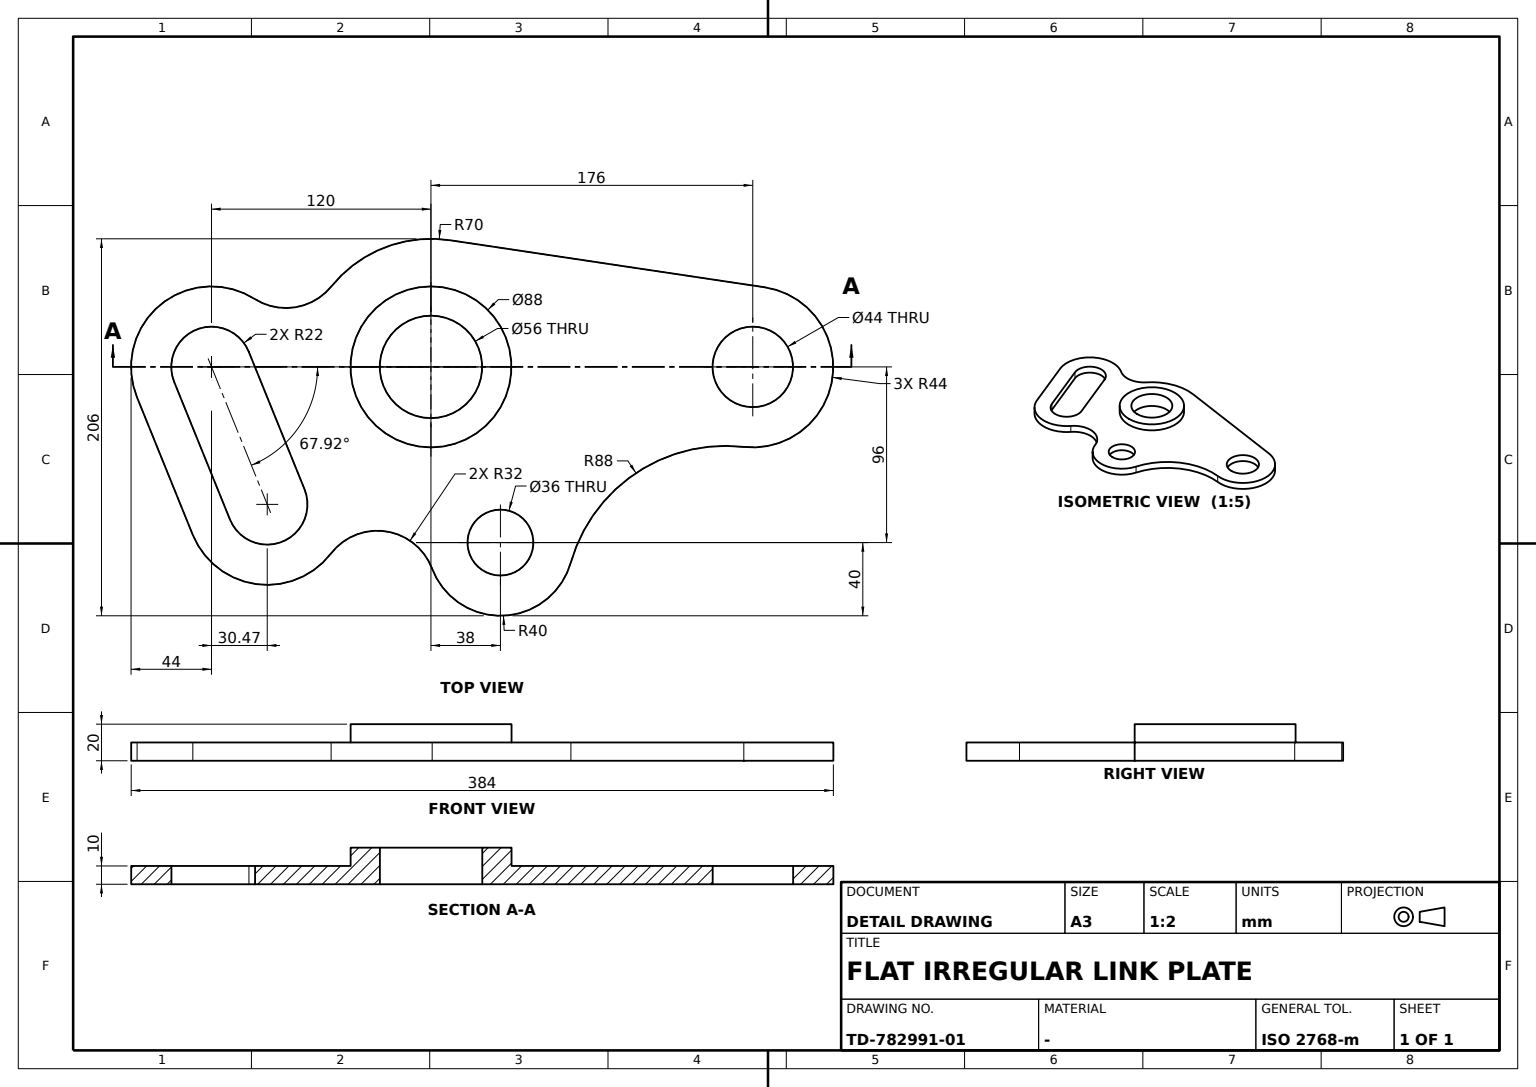
ISO-10303-21;
HEADER;
FILE_DESCRIPTION((''),'2;1');
FILE_NAME('','',(''),(''),'','','');
FILE_SCHEMA(('AUTOMOTIVE_DESIGN'));
ENDSEC;
DATA;
#1=APPLICATION_CONTEXT('');
#2=PRODUCT_CONTEXT('',#1,'mechanical');
#3=PRODUCT('','','',(#2));
#4=PRODUCT_DEFINITION_FORMATION('','',#3);
#5=PRODUCT_DEFINITION_CONTEXT('',#1,'design');
#6=PRODUCT_DEFINITION('','',#4,#5);
#7=PRODUCT_DEFINITION_SHAPE('','',#6);
#8=(LENGTH_UNIT()NAMED_UNIT(*)SI_UNIT(.MILLI.,.METRE.));
#9=(NAMED_UNIT(*)PLANE_ANGLE_UNIT()SI_UNIT($,.RADIAN.));
#10=(NAMED_UNIT(*)SI_UNIT($,.STERADIAN.)SOLID_ANGLE_UNIT());
#11=UNCERTAINTY_MEASURE_WITH_UNIT(LENGTH_MEASURE(0.005),#8,'distance_accuracy_value','');
#12=(GEOMETRIC_REPRESENTATION_CONTEXT(3)GLOBAL_UNCERTAINTY_ASSIGNED_CONTEXT((#11))GLOBAL_UNIT_ASSIGNED_CONTEXT((#8,#9,#10))REPRESENTATION_CONTEXT('',''));
#13=CARTESIAN_POINT('',(-43.517238,182.5,0.));
#14=VERTEX_POINT('',#13);
#15=CARTESIAN_POINT('',(-43.517238,182.5,-10.));
#16=VERTEX_POINT('',#15);
#17=CARTESIAN_POINT('',(-43.517238,182.5,-5.));
#18=DIRECTION('',(0.,0.,1.));
#19=VECTOR('',#18,1000.);
#20=LINE('',#17,#19);
#21=EDGE_CURVE('',#14,#16,#20,.F.);
#22=ORIENTED_EDGE('',*,*,#21,.F.);
#23=CARTESIAN_POINT('',(43.717954,171.026016,0.));
#24=VERTEX_POINT('',#23);
#25=CARTESIAN_POINT('',(0.,176.,0.));
#26=DIRECTION('',(1.,0.,0.));
#27=AXIS2_PLACEMENT_3D('',#25,#18,#26);
#28=CIRCLE('',#27,44.);
#29=EDGE_CURVE('',#24,#14,#28,.T.);
#30=ORIENTED_EDGE('',*,*,#29,.F.);
#31=CARTESIAN_POINT('',(43.717954,171.026016,-10.));
#32=VERTEX_POINT('',#31);
#33=CARTESIAN_POINT('',(43.717954,171.026016,-5.));
#34=LINE('',#33,#19);
#35=EDGE_CURVE('',#24,#32,#34,.F.);
#36=ORIENTED_EDGE('',*,*,#35,.T.);
#37=CARTESIAN_POINT('',(0.,176.,-10.));
#38=AXIS2_PLACEMENT_3D('',#37,#18,#26);
#39=CIRCLE('',#38,44.);
#40=EDGE_CURVE('',#32,#16,#39,.T.);
#41=ORIENTED_EDGE('',*,*,#40,.T.);
#42=EDGE_LOOP('',(#22,#30,#36,#41));
#43=FACE_BOUND('',#42,.T.);
#44=CARTESIAN_POINT('',(0.,176.,-5.));
#45=AXIS2_PLACEMENT_3D('',#44,#18,#26);
#46=CYLINDRICAL_SURFACE('',#45,44.);
#47=ADVANCED_FACE('',(#43),#46,.T.);
#48=CARTESIAN_POINT('',(28.,0.,-10.));
#49=VERTEX_POINT('',#48);
#50=CARTESIAN_POINT('',(0.,0.,-10.));
#51=AXIS2_PLACEMENT_3D('',#50,#18,#26);
#52=CIRCLE('',#51,28.);
#53=EDGE_CURVE('',#49,#49,#52,.T.);
#54=ORIENTED_EDGE('',*,*,#53,.T.);
#55=EDGE_LOOP('',(#54));
#56=FACE_BOUND('',#55,.T.);
#57=CARTESIAN_POINT('',(22.,176.,-10.));
#58=VERTEX_POINT('',#57);
#59=CIRCLE('',#38,22.);
#60=EDGE_CURVE('',#58,#58,#59,.T.);
#61=ORIENTED_EDGE('',*,*,#60,.T.);
#62=EDGE_LOOP('',(#61));
#63=FACE_BOUND('',#62,.T.);
#64=CARTESIAN_POINT('',(-8.270016,-99.613563,-10.));
#65=VERTEX_POINT('',#64);
#66=CARTESIAN_POINT('',(66.851293,-69.139653,-10.));
#67=VERTEX_POINT('',#66);
#68=DIRECTION('',(0.926656248,0.375909827,0.));
#69=VECTOR('',#68,1000.);
#70=LINE('',#64,#69);
#71=EDGE_CURVE('',#65,#67,#70,.T.);
#72=ORIENTED_EDGE('',*,*,#71,.F.);
#73=CARTESIAN_POINT('',(8.270016,-140.386437,-10.));
#74=VERTEX_POINT('',#73);
#75=CARTESIAN_POINT('',(0.,-120.,-10.));
#76=AXIS2_PLACEMENT_3D('',#75,#18,#26);
#77=CIRCLE('',#76,22.);
#78=EDGE_CURVE('',#65,#74,#77,.T.);
#79=ORIENTED_EDGE('',*,*,#78,.T.);
#80=CARTESIAN_POINT('',(83.391326,-109.912528,-10.));
#81=VERTEX_POINT('',#80);
#82=DIRECTION('',(-0.926656248,-0.375909827,0.));
#83=VECTOR('',#82,1000.);
#84=LINE('',#80,#83);
#85=EDGE_CURVE('',#81,#74,#84,.T.);
#86=ORIENTED_EDGE('',*,*,#85,.F.);
#87=CARTESIAN_POINT('',(75.12131,-89.526091,-10.));
#88=AXIS2_PLACEMENT_3D('',#87,#18,#26);
#89=CIRCLE('',#88,22.);
#90=EDGE_CURVE('',#81,#67,#89,.T.);
#91=ORIENTED_EDGE('',*,*,#90,.T.);
#92=EDGE_LOOP('',(#72,#79,#86,#91));
#93=FACE_BOUND('',#92,.T.);
#94=CARTESIAN_POINT('',(-69.231969,10.340909,-10.));
#95=VERTEX_POINT('',#94);
#96=DIRECTION('',(0.147727273,0.989028136,0.));
#97=VECTOR('',#96,1000.);
#98=LINE('',#94,#97);
#99=EDGE_CURVE('',#95,#16,#98,.T.);
#100=ORIENTED_EDGE('',*,*,#99,.T.);
#101=ORIENTED_EDGE('',*,*,#40,.F.);
#102=CARTESIAN_POINT('',(106.985582,76.46189,-10.));
#103=VERTEX_POINT('',#102);
#104=CARTESIAN_POINT('',(131.153861,161.078049,-10.));
#105=AXIS2_PLACEMENT_3D('',#104,#18,#26);
#106=CIRCLE('',#105,88.);
#107=EDGE_CURVE('',#32,#103,#106,.T.);
#108=ORIENTED_EDGE('',*,*,#107,.T.);
#109=CARTESIAN_POINT('',(110.17399,0.595482,-10.));
#110=VERTEX_POINT('',#109);
#111=CARTESIAN_POINT('',(96.,38.,-10.));
#112=AXIS2_PLACEMENT_3D('',#111,#18,#26);
#113=CIRCLE('',#112,40.);
#114=EDGE_CURVE('',#110,#103,#113,.T.);
#115=ORIENTED_EDGE('',*,*,#114,.F.);
#116=CARTESIAN_POINT('',(101.979763,-54.674642,-10.));
#117=VERTEX_POINT('',#116);
#118=CARTESIAN_POINT('',(121.513183,-29.328133,-10.));
#119=AXIS2_PLACEMENT_3D('',#118,#18,#26);
#120=CIRCLE('',#119,32.);
#121=EDGE_CURVE('',#110,#117,#120,.T.);
#122=ORIENTED_EDGE('',*,*,#121,.T.);
#123=CARTESIAN_POINT('',(91.661342,-130.298966,-10.));
#124=VERTEX_POINT('',#123);
#125=CIRCLE('',#88,44.);
#126=EDGE_CURVE('',#124,#117,#125,.T.);
#127=ORIENTED_EDGE('',*,*,#126,.F.);
#128=CARTESIAN_POINT('',(16.540032,-160.772875,-10.));
#129=VERTEX_POINT('',#128);
#130=LINE('',#123,#83);
#131=EDGE_CURVE('',#124,#129,#130,.T.);
#132=ORIENTED_EDGE('',*,*,#131,.T.);
#133=CARTESIAN_POINT('',(-37.152695,-96.427193,-10.));
#134=VERTEX_POINT('',#133);
#135=CIRCLE('',#76,44.);
#136=EDGE_CURVE('',#134,#129,#135,.T.);
#137=ORIENTED_EDGE('',*,*,#136,.F.);
#138=CARTESIAN_POINT('',(-44.040183,-54.410131,-10.));
#139=VERTEX_POINT('',#138);
#140=CARTESIAN_POINT('',(-64.172837,-79.283333,-10.));
#141=AXIS2_PLACEMENT_3D('',#140,#18,#26);
#142=CIRCLE('',#141,32.);
#143=EDGE_CURVE('',#134,#139,#142,.T.);
#144=ORIENTED_EDGE('',*,*,#143,.T.);
#145=CIRCLE('',#51,70.);
#146=EDGE_CURVE('',#95,#139,#145,.T.);
#147=ORIENTED_EDGE('',*,*,#146,.F.);
#148=EDGE_LOOP('',(#100,#101,#108,#115,#122,#127,#132,#137,#144,#147));
#149=FACE_BOUND('',#148,.T.);
#150=CARTESIAN_POINT('',(114.,38.,-10.));
#151=VERTEX_POINT('',#150);
#152=CIRCLE('',#112,18.);
#153=EDGE_CURVE('',#151,#151,#152,.T.);
#154=ORIENTED_EDGE('',*,*,#153,.T.);
#155=EDGE_LOOP('',(#154));
#156=FACE_BOUND('',#155,.T.);
#157=PLANE('',#51);
#158=ADVANCED_FACE('',(#56,#63,#93,#149,#156),#157,.F.);
#159=ORIENTED_EDGE('',*,*,#60,.F.);
#160=EDGE_LOOP('',(#159));
#161=FACE_BOUND('',#160,.T.);
#162=CARTESIAN_POINT('',(22.,176.,0.));
#163=VERTEX_POINT('',#162);
#164=CIRCLE('',#27,22.);
#165=EDGE_CURVE('',#163,#163,#164,.T.);
#166=ORIENTED_EDGE('',*,*,#165,.T.);
#167=EDGE_LOOP('',(#166));
#168=FACE_BOUND('',#167,.T.);
#169=CYLINDRICAL_SURFACE('',#45,22.);
#170=ADVANCED_FACE('',(#161,#168),#169,.F.);
#171=CARTESIAN_POINT('',(28.,0.,10.));
#172=VERTEX_POINT('',#171);
#173=CARTESIAN_POINT('',(0.,0.,10.));
#174=AXIS2_PLACEMENT_3D('',#173,#18,#26);
#175=CIRCLE('',#174,28.);
#176=EDGE_CURVE('',#172,#172,#175,.T.);
#177=ORIENTED_EDGE('',*,*,#176,.T.);
#178=EDGE_LOOP('',(#177));
#179=FACE_BOUND('',#178,.T.);
#180=ORIENTED_EDGE('',*,*,#53,.F.);
#181=EDGE_LOOP('',(#180));
#182=FACE_BOUND('',#181,.T.);
#183=CARTESIAN_POINT('',(0.,0.,-5.));
#184=AXIS2_PLACEMENT_3D('',#183,#18,#26);
#185=CYLINDRICAL_SURFACE('',#184,28.);
#186=ADVANCED_FACE('',(#179,#182),#185,.F.);
#187=CARTESIAN_POINT('',(66.851293,-69.139653,0.));
#188=VERTEX_POINT('',#187);
#189=CARTESIAN_POINT('',(66.851293,-69.139653,-5.));
#190=LINE('',#189,#19);
#191=EDGE_CURVE('',#188,#67,#190,.F.);
#192=ORIENTED_EDGE('',*,*,#191,.F.);
#193=CARTESIAN_POINT('',(-8.270016,-99.613563,0.));
#194=VERTEX_POINT('',#193);
#195=LINE('',#193,#69);
#196=EDGE_CURVE('',#194,#188,#195,.T.);
#197=ORIENTED_EDGE('',*,*,#196,.F.);
#198=CARTESIAN_POINT('',(-8.270016,-99.613563,-5.));
#199=LINE('',#198,#19);
#200=EDGE_CURVE('',#194,#65,#199,.F.);
#201=ORIENTED_EDGE('',*,*,#200,.T.);
#202=ORIENTED_EDGE('',*,*,#71,.T.);
#203=EDGE_LOOP('',(#192,#197,#201,#202));
#204=FACE_BOUND('',#203,.T.);
#205=DIRECTION('',(-0.375909827,0.926656248,0.));
#206=AXIS2_PLACEMENT_3D('',#193,#205,#68);
#207=PLANE('',#206);
#208=ADVANCED_FACE('',(#204),#207,.F.);
#209=CARTESIAN_POINT('',(83.391326,-109.912528,0.));
#210=VERTEX_POINT('',#209);
#211=CARTESIAN_POINT('',(75.12131,-89.526091,0.));
#212=AXIS2_PLACEMENT_3D('',#211,#18,#26);
#213=CIRCLE('',#212,22.);
#214=EDGE_CURVE('',#210,#188,#213,.T.);
#215=ORIENTED_EDGE('',*,*,#214,.T.);
#216=ORIENTED_EDGE('',*,*,#191,.T.);
#217=ORIENTED_EDGE('',*,*,#90,.F.);
#218=CARTESIAN_POINT('',(83.391326,-109.912528,-5.));
#219=LINE('',#218,#19);
#220=EDGE_CURVE('',#210,#81,#219,.F.);
#221=ORIENTED_EDGE('',*,*,#220,.F.);
#222=EDGE_LOOP('',(#215,#216,#217,#221));
#223=FACE_BOUND('',#222,.T.);
#224=CARTESIAN_POINT('',(75.12131,-89.526091,-5.));
#225=AXIS2_PLACEMENT_3D('',#224,#18,#26);
#226=CYLINDRICAL_SURFACE('',#225,22.);
#227=ADVANCED_FACE('',(#223),#226,.F.);
#228=ORIENTED_EDGE('',*,*,#200,.F.);
#229=CARTESIAN_POINT('',(8.270016,-140.386437,0.));
#230=VERTEX_POINT('',#229);
#231=CARTESIAN_POINT('',(0.,-120.,0.));
#232=AXIS2_PLACEMENT_3D('',#231,#18,#26);
#233=CIRCLE('',#232,22.);
#234=EDGE_CURVE('',#194,#230,#233,.T.);
#235=ORIENTED_EDGE('',*,*,#234,.T.);
#236=CARTESIAN_POINT('',(8.270016,-140.386437,-5.));
#237=LINE('',#236,#19);
#238=EDGE_CURVE('',#230,#74,#237,.F.);
#239=ORIENTED_EDGE('',*,*,#238,.T.);
#240=ORIENTED_EDGE('',*,*,#78,.F.);
#241=EDGE_LOOP('',(#228,#235,#239,#240));
#242=FACE_BOUND('',#241,.T.);
#243=CARTESIAN_POINT('',(0.,-120.,-5.));
#244=AXIS2_PLACEMENT_3D('',#243,#18,#26);
#245=CYLINDRICAL_SURFACE('',#244,22.);
#246=ADVANCED_FACE('',(#242),#245,.F.);
#247=ORIENTED_EDGE('',*,*,#21,.T.);
#248=ORIENTED_EDGE('',*,*,#99,.F.);
#249=CARTESIAN_POINT('',(-69.231969,10.340909,0.));
#250=VERTEX_POINT('',#249);
#251=CARTESIAN_POINT('',(-69.231969,10.340909,-5.));
#252=LINE('',#251,#19);
#253=EDGE_CURVE('',#250,#95,#252,.F.);
#254=ORIENTED_EDGE('',*,*,#253,.F.);
#255=LINE('',#249,#97);
#256=EDGE_CURVE('',#250,#14,#255,.T.);
#257=ORIENTED_EDGE('',*,*,#256,.T.);
#258=EDGE_LOOP('',(#247,#248,#254,#257));
#259=FACE_BOUND('',#258,.T.);
#260=DIRECTION('',(-0.989028136,0.147727273,0.));
#261=AXIS2_PLACEMENT_3D('',#249,#260,#96);
#262=PLANE('',#261);
#263=ADVANCED_FACE('',(#259),#262,.T.);
#264=CARTESIAN_POINT('',(16.540032,-160.772875,0.));
#265=VERTEX_POINT('',#264);
#266=CARTESIAN_POINT('',(16.540032,-160.772875,-5.));
#267=LINE('',#266,#19);
#268=EDGE_CURVE('',#265,#129,#267,.F.);
#269=ORIENTED_EDGE('',*,*,#268,.T.);
#270=ORIENTED_EDGE('',*,*,#131,.F.);
#271=CARTESIAN_POINT('',(91.661342,-130.298966,0.));
#272=VERTEX_POINT('',#271);
#273=CARTESIAN_POINT('',(91.661342,-130.298966,-5.));
#274=LINE('',#273,#19);
#275=EDGE_CURVE('',#272,#124,#274,.F.);
#276=ORIENTED_EDGE('',*,*,#275,.F.);
#277=LINE('',#271,#83);
#278=EDGE_CURVE('',#272,#265,#277,.T.);
#279=ORIENTED_EDGE('',*,*,#278,.T.);
#280=EDGE_LOOP('',(#269,#270,#276,#279));
#281=FACE_BOUND('',#280,.T.);
#282=DIRECTION('',(0.375909827,-0.926656248,0.));
#283=AXIS2_PLACEMENT_3D('',#271,#282,#82);
#284=PLANE('',#283);
#285=ADVANCED_FACE('',(#281),#284,.T.);
#286=ORIENTED_EDGE('',*,*,#85,.T.);
#287=ORIENTED_EDGE('',*,*,#238,.F.);
#288=LINE('',#209,#83);
#289=EDGE_CURVE('',#210,#230,#288,.T.);
#290=ORIENTED_EDGE('',*,*,#289,.F.);
#291=ORIENTED_EDGE('',*,*,#220,.T.);
#292=EDGE_LOOP('',(#286,#287,#290,#291));
#293=FACE_BOUND('',#292,.T.);
#294=AXIS2_PLACEMENT_3D('',#209,#282,#82);
#295=PLANE('',#294);
#296=ADVANCED_FACE('',(#293),#295,.F.);
#297=CARTESIAN_POINT('',(110.17399,0.595482,0.));
#298=VERTEX_POINT('',#297);
#299=CARTESIAN_POINT('',(101.979763,-54.674642,0.));
#300=VERTEX_POINT('',#299);
#301=CARTESIAN_POINT('',(121.513183,-29.328133,0.));
#302=AXIS2_PLACEMENT_3D('',#301,#18,#26);
#303=CIRCLE('',#302,32.);
#304=EDGE_CURVE('',#298,#300,#303,.T.);
#305=ORIENTED_EDGE('',*,*,#304,.T.);
#306=CARTESIAN_POINT('',(101.979763,-54.674642,-5.));
#307=LINE('',#306,#19);
#308=EDGE_CURVE('',#300,#117,#307,.F.);
#309=ORIENTED_EDGE('',*,*,#308,.T.);
#310=ORIENTED_EDGE('',*,*,#121,.F.);
#311=CARTESIAN_POINT('',(110.17399,0.595482,-5.));
#312=LINE('',#311,#19);
#313=EDGE_CURVE('',#298,#110,#312,.F.);
#314=ORIENTED_EDGE('',*,*,#313,.F.);
#315=EDGE_LOOP('',(#305,#309,#310,#314));
#316=FACE_BOUND('',#315,.T.);
#317=CARTESIAN_POINT('',(121.513183,-29.328133,-5.));
#318=AXIS2_PLACEMENT_3D('',#317,#18,#26);
#319=CYLINDRICAL_SURFACE('',#318,32.);
#320=ADVANCED_FACE('',(#316),#319,.F.);
#321=CARTESIAN_POINT('',(106.985582,76.46189,0.));
#322=VERTEX_POINT('',#321);
#323=CARTESIAN_POINT('',(131.153861,161.078049,0.));
#324=AXIS2_PLACEMENT_3D('',#323,#18,#26);
#325=CIRCLE('',#324,88.);
#326=EDGE_CURVE('',#24,#322,#325,.T.);
#327=ORIENTED_EDGE('',*,*,#326,.T.);
#328=CARTESIAN_POINT('',(106.985582,76.46189,-5.));
#329=LINE('',#328,#19);
#330=EDGE_CURVE('',#322,#103,#329,.F.);
#331=ORIENTED_EDGE('',*,*,#330,.T.);
#332=ORIENTED_EDGE('',*,*,#107,.F.);
#333=ORIENTED_EDGE('',*,*,#35,.F.);
#334=EDGE_LOOP('',(#327,#331,#332,#333));
#335=FACE_BOUND('',#334,.T.);
#336=CARTESIAN_POINT('',(131.153861,161.078049,-5.));
#337=AXIS2_PLACEMENT_3D('',#336,#18,#26);
#338=CYLINDRICAL_SURFACE('',#337,88.);
#339=ADVANCED_FACE('',(#335),#338,.F.);
#340=ORIENTED_EDGE('',*,*,#126,.T.);
#341=ORIENTED_EDGE('',*,*,#308,.F.);
#342=CIRCLE('',#212,44.);
#343=EDGE_CURVE('',#272,#300,#342,.T.);
#344=ORIENTED_EDGE('',*,*,#343,.F.);
#345=ORIENTED_EDGE('',*,*,#275,.T.);
#346=EDGE_LOOP('',(#340,#341,#344,#345));
#347=FACE_BOUND('',#346,.T.);
#348=CYLINDRICAL_SURFACE('',#225,44.);
#349=ADVANCED_FACE('',(#347),#348,.T.);
#350=ORIENTED_EDGE('',*,*,#29,.T.);
#351=ORIENTED_EDGE('',*,*,#256,.F.);
#352=CARTESIAN_POINT('',(-44.040183,-54.410131,0.));
#353=VERTEX_POINT('',#352);
#354=CARTESIAN_POINT('',(0.,0.,0.));
#355=AXIS2_PLACEMENT_3D('',#354,#18,#26);
#356=CIRCLE('',#355,70.);
#357=EDGE_CURVE('',#250,#353,#356,.T.);
#358=ORIENTED_EDGE('',*,*,#357,.T.);
#359=CARTESIAN_POINT('',(-37.152695,-96.427193,0.));
#360=VERTEX_POINT('',#359);
#361=CARTESIAN_POINT('',(-64.172837,-79.283333,0.));
#362=AXIS2_PLACEMENT_3D('',#361,#18,#26);
#363=CIRCLE('',#362,32.);
#364=EDGE_CURVE('',#360,#353,#363,.T.);
#365=ORIENTED_EDGE('',*,*,#364,.F.);
#366=CIRCLE('',#232,44.);
#367=EDGE_CURVE('',#360,#265,#366,.T.);
#368=ORIENTED_EDGE('',*,*,#367,.T.);
#369=ORIENTED_EDGE('',*,*,#278,.F.);
#370=ORIENTED_EDGE('',*,*,#343,.T.);
#371=ORIENTED_EDGE('',*,*,#304,.F.);
#372=CARTESIAN_POINT('',(96.,38.,0.));
#373=AXIS2_PLACEMENT_3D('',#372,#18,#26);
#374=CIRCLE('',#373,40.);
#375=EDGE_CURVE('',#298,#322,#374,.T.);
#376=ORIENTED_EDGE('',*,*,#375,.T.);
#377=ORIENTED_EDGE('',*,*,#326,.F.);
#378=EDGE_LOOP('',(#350,#351,#358,#365,#368,#369,#370,#371,#376,#377));
#379=FACE_BOUND('',#378,.T.);
#380=ORIENTED_EDGE('',*,*,#165,.F.);
#381=EDGE_LOOP('',(#380));
#382=FACE_BOUND('',#381,.T.);
#383=CARTESIAN_POINT('',(44.,0.,0.));
#384=VERTEX_POINT('',#383);
#385=CIRCLE('',#355,44.);
#386=EDGE_CURVE('',#384,#384,#385,.T.);
#387=ORIENTED_EDGE('',*,*,#386,.F.);
#388=EDGE_LOOP('',(#387));
#389=FACE_BOUND('',#388,.T.);
#390=ORIENTED_EDGE('',*,*,#234,.F.);
#391=ORIENTED_EDGE('',*,*,#196,.T.);
#392=ORIENTED_EDGE('',*,*,#214,.F.);
#393=ORIENTED_EDGE('',*,*,#289,.T.);
#394=EDGE_LOOP('',(#390,#391,#392,#393));
#395=FACE_BOUND('',#394,.T.);
#396=CARTESIAN_POINT('',(114.,38.,0.));
#397=VERTEX_POINT('',#396);
#398=CIRCLE('',#373,18.);
#399=EDGE_CURVE('',#397,#397,#398,.T.);
#400=ORIENTED_EDGE('',*,*,#399,.F.);
#401=EDGE_LOOP('',(#400));
#402=FACE_BOUND('',#401,.T.);
#403=PLANE('',#355);
#404=ADVANCED_FACE('',(#379,#382,#389,#395,#402),#403,.T.);
#405=ORIENTED_EDGE('',*,*,#153,.F.);
#406=EDGE_LOOP('',(#405));
#407=FACE_BOUND('',#406,.T.);
#408=ORIENTED_EDGE('',*,*,#399,.T.);
#409=EDGE_LOOP('',(#408));
#410=FACE_BOUND('',#409,.T.);
#411=CARTESIAN_POINT('',(96.,38.,-5.));
#412=AXIS2_PLACEMENT_3D('',#411,#18,#26);
#413=CYLINDRICAL_SURFACE('',#412,18.);
#414=ADVANCED_FACE('',(#407,#410),#413,.F.);
#415=CARTESIAN_POINT('',(44.,0.,10.));
#416=VERTEX_POINT('',#415);
#417=CIRCLE('',#174,44.);
#418=EDGE_CURVE('',#416,#416,#417,.T.);
#419=ORIENTED_EDGE('',*,*,#418,.T.);
#420=EDGE_LOOP('',(#419));
#421=FACE_BOUND('',#420,.T.);
#422=ORIENTED_EDGE('',*,*,#176,.F.);
#423=EDGE_LOOP('',(#422));
#424=FACE_BOUND('',#423,.T.);
#425=PLANE('',#174);
#426=ADVANCED_FACE('',(#421,#424),#425,.T.);
#427=ORIENTED_EDGE('',*,*,#268,.F.);
#428=ORIENTED_EDGE('',*,*,#367,.F.);
#429=CARTESIAN_POINT('',(-37.152695,-96.427193,-5.));
#430=LINE('',#429,#19);
#431=EDGE_CURVE('',#360,#134,#430,.F.);
#432=ORIENTED_EDGE('',*,*,#431,.T.);
#433=ORIENTED_EDGE('',*,*,#136,.T.);
#434=EDGE_LOOP('',(#427,#428,#432,#433));
#435=FACE_BOUND('',#434,.T.);
#436=CYLINDRICAL_SURFACE('',#244,44.);
#437=ADVANCED_FACE('',(#435),#436,.T.);
#438=ORIENTED_EDGE('',*,*,#418,.F.);
#439=EDGE_LOOP('',(#438));
#440=FACE_BOUND('',#439,.T.);
#441=ORIENTED_EDGE('',*,*,#386,.T.);
#442=EDGE_LOOP('',(#441));
#443=FACE_BOUND('',#442,.T.);
#444=CARTESIAN_POINT('',(0.,0.,5.));
#445=AXIS2_PLACEMENT_3D('',#444,#18,#26);
#446=CYLINDRICAL_SURFACE('',#445,44.);
#447=ADVANCED_FACE('',(#440,#443),#446,.T.);
#448=CARTESIAN_POINT('',(-44.040183,-54.410131,-5.));
#449=LINE('',#448,#19);
#450=EDGE_CURVE('',#353,#139,#449,.F.);
#451=ORIENTED_EDGE('',*,*,#450,.T.);
#452=ORIENTED_EDGE('',*,*,#143,.F.);
#453=ORIENTED_EDGE('',*,*,#431,.F.);
#454=ORIENTED_EDGE('',*,*,#364,.T.);
#455=EDGE_LOOP('',(#451,#452,#453,#454));
#456=FACE_BOUND('',#455,.T.);
#457=CARTESIAN_POINT('',(-64.172837,-79.283333,-5.));
#458=AXIS2_PLACEMENT_3D('',#457,#18,#26);
#459=CYLINDRICAL_SURFACE('',#458,32.);
#460=ADVANCED_FACE('',(#456),#459,.F.);
#461=ORIENTED_EDGE('',*,*,#330,.F.);
#462=ORIENTED_EDGE('',*,*,#375,.F.);
#463=ORIENTED_EDGE('',*,*,#313,.T.);
#464=ORIENTED_EDGE('',*,*,#114,.T.);
#465=EDGE_LOOP('',(#461,#462,#463,#464));
#466=FACE_BOUND('',#465,.T.);
#467=CYLINDRICAL_SURFACE('',#412,40.);
#468=ADVANCED_FACE('',(#466),#467,.T.);
#469=ORIENTED_EDGE('',*,*,#146,.T.);
#470=ORIENTED_EDGE('',*,*,#450,.F.);
#471=ORIENTED_EDGE('',*,*,#357,.F.);
#472=ORIENTED_EDGE('',*,*,#253,.T.);
#473=EDGE_LOOP('',(#469,#470,#471,#472));
#474=FACE_BOUND('',#473,.T.);
#475=CYLINDRICAL_SURFACE('',#184,70.);
#476=ADVANCED_FACE('',(#474),#475,.T.);
#477=CLOSED_SHELL('',(#47,#158,#170,#186,#208,#227,#246,#263,#285,#296,#320,#339,#349,#404,#414,#426,#437,#447,#460,#468,#476));
#478=MANIFOLD_SOLID_BREP('',#477);
#479=ADVANCED_BREP_SHAPE_REPRESENTATION('',(#478),#12);
#480=SHAPE_DEFINITION_REPRESENTATION(#7,#479);
ENDSEC;
END-ISO-10303-21;
